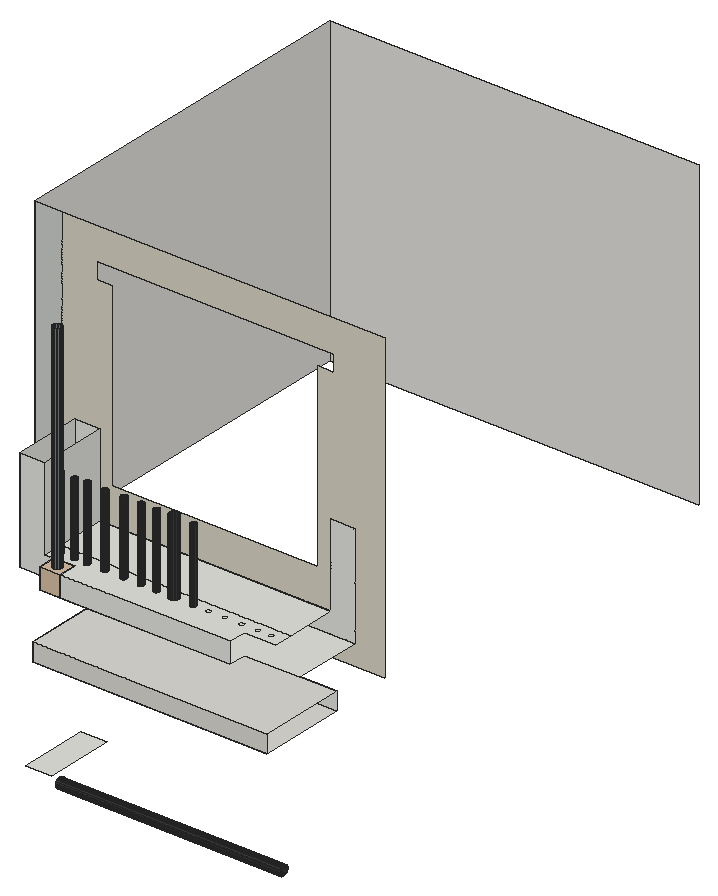
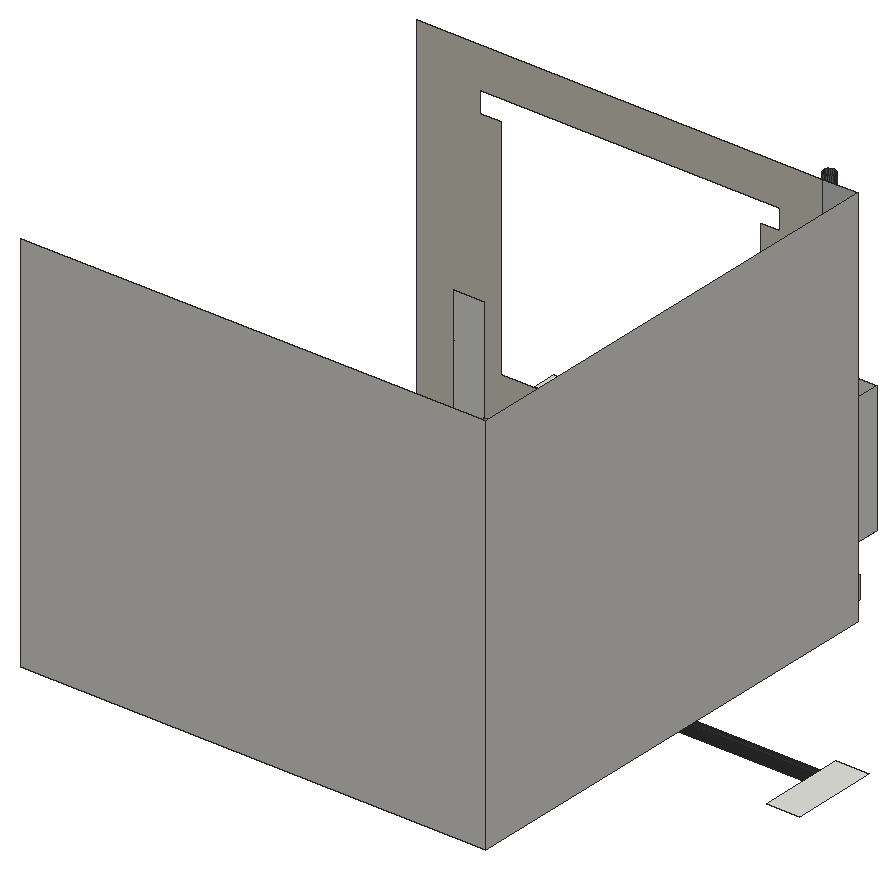
# SketchUp Ruby script. Lengths in inches.
U = 1.inch
M = Sketchup.active_model
def pt(a) = Geom::Point3d.new(a.map { |v| v * U })
def face(e, loops, mat)
  f = e.add_face(loops[0].map { |a| pt(a) })
  loops[1..].each { |l| e.add_face(l.map { |a| pt(a) }).erase! }
  f.material = f.back_material = mat if mat
  f
end
# faces: each face lists its corners as indices into pts; further lists are holes
def faces(e, pts, list, mat = nil) = list.each { |f| face(e, (f[0].is_a?(Array) ? f : [f]).map { |l| l.map { |i| pts[i] } }, mat) }
# xy, xz, yz: faces in a plane at the given z, y or x. An outline is a flat list of corners, or four numbers for a rectangle; further outlines are holes
def ring(l) = l.size == 4 ? [[l[0], l[1]], [l[2], l[1]], [l[2], l[3]], [l[0], l[3]]] : l.each_slice(2).to_a
def flat(e, list, mat, &to3) = list.each { |f| face(e, (f[0].is_a?(Array) ? f : [f]).map { |l| ring(l).map { |u, v| to3.(u, v) } }, mat) }
def xy(e, z, list, mat = nil) = flat(e, list, mat) { |x, y| [x, y, z] }
def xz(e, y, list, mat = nil) = flat(e, list, mat) { |x, z| [x, y, z] }
def yz(e, x, list, mat = nil) = flat(e, list, mat) { |y, z| [x, y, z] }
def lines(e, pts, list) = list.each { |a, b| e.add_line(pt(pts[a]), pt(pts[b])) }
# prism: a flat outline (further loops are holes) pulled along v
def prism(e, loops, v, mat = nil)
  f = face(e, loops, mat); d = Geom::Vector3d.new(v.map { |x| x * U })
  f.pushpull(f.normal.samedirection?(d) ? d.length : -d.length)
end
def box(e, o, s, mat = nil) = prism(e, [[o, [o[0] + s[0], o[1], o[2]], [o[0] + s[0], o[1] + s[1], o[2]], [o[0], o[1] + s[1], o[2]]]], [0, 0, s[2]], mat)
def at(x, y, z, deg = 0) = Geom::Transformation.translation(pt([x, y, z])) * Geom::Transformation.rotation(ORIGIN, Z_AXIS, deg.degrees)
def axes(o, x, y, z) = Geom::Transformation.new([*x, 0, *y, 0, *z, 0, *pt(o).to_a, 1])
def part(name) = M.definitions.add(name)
# library, detail: a bought-in or finely detailed component or shape, given as its bounding box
def library(name, o, s) = part(name).tap { |d| box(d.entities, o, s) }
def detail(e, o, s) = box(e.add_group.entities, o, s)
def put(e, d, t, mat = nil) = e.add_instance(d, t).tap { |i| i.material = mat if mat }
def group(e, t, mat = nil) = e.add_group.tap { |g| g.transformation = t; g.material = mat if mat }.entities
root = M.entities
M.materials.add("[Basic Tile]").color = [203, 206, 202]
M.materials.add("[Color M07]").color = [58, 58, 58]
M.materials.add("[Formica Graystone]1").color = [216, 212, 196]
M.materials.add("[Formica Laminate Light]").color = [213, 189, 164]
M.materials.add("[Formica Speckled Grey]").color = [112, 125, 132]
M.materials.add("[Quartz Light Brown]").color = [199, 184, 152]
M.materials.add("[Terrazzo Tile Accent]").color = [224, 221, 217]
M.materials.add("[Terrazzo Tile Light]").color = [219, 217, 210]
xy(root,298.58,[[85.8,91.86,86.02,91.89,86.24,91.97,86.42,92.11,86.56,92.29,86.64,92.5,86.67,92.73,86.64,92.96,86.56,93.17,86.42,93.35,86.24,93.49,86.02,93.58,85.8,93.61,85.57,93.58,85.36,93.49,85.18,93.35,85.04,93.17,84.95,92.96,84.92,92.73,84.95,92.5,85.04,92.29,85.18,92.11,85.36,91.97,85.57,91.89]])
xy(root,298.77,[[73.9,91.87,74.08,91.89,74.25,91.96,74.39,92.07,74.5,92.21,74.57,92.38,74.59,92.56,74.57,92.73,74.5,92.9,74.39,93.04,74.25,93.15,74.08,93.22,73.9,93.24,73.73,93.22,73.5625,93.15,73.42,93.04,73.31,92.9,73.24,92.73,73.22,92.56,73.24,92.38,73.31,92.21,73.42,92.07,73.5625,91.96,73.73,91.89]])
xy(root,299.33,[[67.78,91.87,67.96,91.89,68.125,91.96,68.27,92.07,68.375,92.21,68.44,92.38,68.47,92.56,68.44,92.73,68.375,92.9,68.27,93.04,68.125,93.15,67.96,93.22,67.78,93.24,67.6,93.22,67.4375,93.15,67.29,93.04,67.18,92.9,67.12,92.73,67.09,92.56,67.12,92.38,67.18,92.21,67.29,92.07,67.4375,91.96,67.6,91.89]])
xy(root,299.71,[[50.09,91.87,50.27,91.89,50.4375,91.96,50.58,92.07,50.6875,92.21,50.76,92.38,50.78,92.56,50.76,92.73,50.6875,92.9,50.58,93.04,50.4375,93.15,50.27,93.22,50.09,93.24,49.91,93.22,49.75,93.15,49.61,93.04,49.5,92.9,49.43,92.73,49.4,92.56,49.43,92.38,49.5,92.21,49.61,92.07,49.75,91.96,49.91,91.89]])
xy(root,299.74,[[55.47,91.87,55.64,91.89,55.8125,91.96,55.95,92.07,56.0625,92.21,56.13,92.38,56.15,92.56,56.13,92.73,56.0625,92.9,55.95,93.04,55.8125,93.15,55.64,93.22,55.47,93.24,55.29,93.22,55.125,93.15,54.98,93.04,54.87,92.9,54.8,92.73,54.78,92.56,54.8,92.38,54.87,92.21,54.98,92.07,55.125,91.96,55.29,91.89],[61.72,91.87,61.89,91.89,62.0625,91.96,62.2,92.07,62.3125,92.21,62.38,92.38,62.4,92.56,62.38,92.73,62.3125,92.9,62.2,93.04,62.0625,93.15,61.89,93.22,61.72,93.24,61.54,93.22,61.375,93.15,61.23,93.04,61.12,92.9,61.05,92.73,61.03,92.56,61.05,92.38,61.12,92.21,61.23,92.07,61.375,91.96,61.54,91.89],[80.03,91.87,80.21,91.89,80.375,91.96,80.52,92.07,80.625,92.21,80.69,92.38,80.72,92.56,80.69,92.73,80.625,92.9,80.52,93.04,80.375,93.15,80.21,93.22,80.03,93.24,79.85,93.22,79.6875,93.15,79.54,93.04,79.43,92.9,79.37,92.73,79.34,92.56,79.37,92.38,79.43,92.21,79.54,92.07,79.6875,91.96,79.85,91.89],[90.97,91.87,91.14,91.89,91.3125,91.96,91.45,92.07,91.5625,92.21,91.63,92.38,91.65,92.56,91.63,92.73,91.5625,92.9,91.45,93.04,91.3125,93.15,91.14,93.22,90.97,93.24,90.79,93.22,90.625,93.15,90.48,93.04,90.37,92.9,90.3,92.73,90.28,92.56,90.3,92.38,90.37,92.21,90.48,92.07,90.625,91.96,90.79,91.89]])
xy(root,302.83,[[37.87,89.73,47.16,114.1]])
xy(root,338.67,[[51.12,107.85,119.37,114.1]],"[Quartz Light Brown]")
xy(root,339.99,[[51.12,107.85,119.37,109.1],[51.12,109.1,119.37,114.1]])
xy(root,341.31,[[51.12,109.1,119.37,114.1]])
xy(root,341.31,[[[45.36,83.35,45.36,114.1,51.12,114.1,51.12,109.1,119.37,109.1,119.37,114.1,128.55,114.1,128.55,83.35],[120.4,84.29,120.93,84.36,121.43,84.57,121.86,84.89,122.18,85.32,122.39,85.82,122.46,86.35,122.39,86.89,122.18,87.38,121.86,87.8125,121.43,88.14,120.93,88.35,120.4,88.42,119.86,88.35,119.37,88.14,118.9375,87.8125,118.61,87.38,118.41,86.89,118.33,86.35,118.41,85.82,118.61,85.32,118.9375,84.89,119.37,84.57,119.86,84.36],[54.33,84.29,54.87,84.36,55.37,84.57,55.79,84.89,56.12,85.32,56.33,85.82,56.4,86.35,56.33,86.89,56.12,87.38,55.79,87.8125,55.37,88.14,54.87,88.35,54.33,88.42,53.8,88.35,53.3,88.14,52.875,87.8125,52.55,87.38,52.34,86.89,52.27,86.35,52.34,85.82,52.55,85.32,52.875,84.89,53.3,84.57,53.8,84.36]]],"[Terrazzo Tile Light]")
xy(root,347.68,[[45.36,83.35,128.55,114.1]],"[Terrazzo Tile Light]")
xy(root,365.02,[[55.11,83.42,55.11,89.73,35.74,89.73,35.74,114.1,135.17,114.1,135.17,89.73,115.36,89.73,115.36,83.42]])
xy(root,365.02,[[47.86,83.42,55.11,89.73]],"[Formica Laminate Light]")
xy(root,372.27,[[[55.11,83.42,115.36,83.42,115.36,89.73,126.56,89.73,126.56,96.33,44.74,96.33,44.74,89.73,55.11,89.73],[87.78,91.42,87.36,91.47,86.97,91.63,86.63,91.89,86.375,92.23,86.21,92.62,86.16,93.04,86.21,93.46,86.375,93.85,86.63,94.19,86.97,94.45,87.36,94.61,87.78,94.67,88.2,94.61,88.59,94.45,88.93,94.19,89.1875,93.85,89.35,93.46,89.41,93.04,89.35,92.62,89.1875,92.23,88.93,91.89,88.59,91.63,88.2,91.47],[94.65,92.0625,94.39,92.1,94.15,92.2,93.94,92.35,93.78,92.5625,93.68,92.8,93.65,93.0625,93.68,93.32,93.78,93.5625,93.94,93.77,94.15,93.93,94.39,94.03,94.65,94.0625,94.91,94.03,95.15,93.93,95.36,93.77,95.52,93.5625,95.62,93.32,95.65,93.0625,95.62,92.8,95.52,92.5625,95.36,92.35,95.15,92.2,94.91,92.1],[122.21,92.0625,121.95,92.1,121.71,92.2,121.5,92.35,121.35,92.5625,121.25,92.8,121.21,93.0625,121.25,93.32,121.35,93.5625,121.5,93.77,121.71,93.93,121.95,94.03,122.21,94.0625,122.47,94.03,122.71,93.93,122.92,93.77,123.08,93.5625,123.18,93.32,123.21,93.0625,123.18,92.8,123.08,92.5625,122.92,92.35,122.71,92.2,122.47,92.1],[100.02,92.0625,99.77,92.1,99.52,92.2,99.32,92.35,99.16,92.5625,99.06,92.8,99.02,93.0625,99.06,93.32,99.16,93.5625,99.32,93.77,99.52,93.93,99.77,94.03,100.02,94.0625,100.28,94.03,100.52,93.93,100.73,93.77,100.89,93.5625,100.99,93.32,101.02,93.0625,100.99,92.8,100.89,92.5625,100.73,92.35,100.52,92.2,100.28,92.1],[117.4,92.0625,117.14,92.1,116.9,92.2,116.69,92.35,116.53,92.5625,116.43,92.8,116.4,93.0625,116.43,93.32,116.53,93.5625,116.69,93.77,116.9,93.93,117.14,94.03,117.4,94.0625,117.66,94.03,117.9,93.93,118.11,93.77,118.27,93.5625,118.37,93.32,118.4,93.0625,118.37,92.8,118.27,92.5625,118.11,92.35,117.9,92.2,117.66,92.1],[105.71,92.0625,105.45,92.1,105.21,92.2,105,92.35,104.85,92.5625,104.75,92.8,104.71,93.0625,104.75,93.32,104.85,93.5625,105,93.77,105.21,93.93,105.45,94.03,105.71,94.0625,105.97,94.03,106.21,93.93,106.42,93.77,106.58,93.5625,106.68,93.32,106.71,93.0625,106.68,92.8,106.58,92.5625,106.42,92.35,106.21,92.2,105.97,92.1],[111.77,92.0625,111.52,92.1,111.27,92.2,111.07,92.35,110.91,92.5625,110.81,92.8,110.77,93.0625,110.81,93.32,110.91,93.5625,111.07,93.77,111.27,93.93,111.52,94.03,111.77,94.0625,112.03,94.03,112.27,93.93,112.48,93.77,112.64,93.5625,112.74,93.32,112.77,93.0625,112.74,92.8,112.64,92.5625,112.48,92.35,112.27,92.2,112.03,92.1],[47.34,92.0625,47.08,92.1,46.84,92.2,46.63,92.35,46.47,92.5625,46.37,92.8,46.34,93.0625,46.37,93.32,46.47,93.5625,46.63,93.77,46.84,93.93,47.08,94.03,47.34,94.0625,47.6,94.03,47.84,93.93,48.04,93.77,48.2,93.5625,48.3,93.32,48.34,93.0625,48.3,92.8,48.2,92.5625,48.04,92.35,47.84,92.2,47.6,92.1],[81.59,92.0625,81.33,92.1,81.09,92.2,80.88,92.35,80.72,92.5625,80.62,92.8,80.59,93.0625,80.62,93.32,80.72,93.5625,80.88,93.77,81.09,93.93,81.33,94.03,81.59,94.0625,81.85,94.03,82.09,93.93,82.29,93.77,82.45,93.5625,82.55,93.32,82.59,93.0625,82.55,92.8,82.45,92.5625,82.29,92.35,82.09,92.2,81.85,92.1],[52.52,92.0625,52.27,92.1,52.02,92.2,51.82,92.35,51.66,92.5625,51.56,92.8,51.52,93.0625,51.56,93.32,51.66,93.5625,51.82,93.77,52.02,93.93,52.27,94.03,52.52,94.0625,52.78,94.03,53.02,93.93,53.23,93.77,53.39,93.5625,53.49,93.32,53.52,93.0625,53.49,92.8,53.39,92.5625,53.23,92.35,53.02,92.2,52.78,92.1],[76.09,92.0625,75.83,92.1,75.59,92.2,75.38,92.35,75.22,92.5625,75.12,92.8,75.09,93.0625,75.12,93.32,75.22,93.5625,75.38,93.77,75.59,93.93,75.83,94.03,76.09,94.0625,76.35,94.03,76.59,93.93,76.79,93.77,76.95,93.5625,77.05,93.32,77.09,93.0625,77.05,92.8,76.95,92.5625,76.79,92.35,76.59,92.2,76.35,92.1],[56.96,92.0625,56.7,92.1,56.46,92.2,56.25,92.35,56.1,92.5625,56,92.8,55.96,93.0625,56,93.32,56.1,93.5625,56.25,93.77,56.46,93.93,56.7,94.03,56.96,94.0625,57.22,94.03,57.46,93.93,57.67,93.77,57.83,93.5625,57.93,93.32,57.96,93.0625,57.93,92.8,57.83,92.5625,57.67,92.35,57.46,92.2,57.22,92.1],[69.96,92.0625,69.7,92.1,69.46,92.2,69.25,92.35,69.1,92.5625,69,92.8,68.96,93.0625,69,93.32,69.1,93.5625,69.25,93.77,69.46,93.93,69.7,94.03,69.96,94.0625,70.22,94.03,70.46,93.93,70.67,93.77,70.83,93.5625,70.93,93.32,70.96,93.0625,70.93,92.8,70.83,92.5625,70.67,92.35,70.46,92.2,70.22,92.1],[63.21,92.0625,62.95,92.1,62.71,92.2,62.5,92.35,62.35,92.5625,62.25,92.8,62.21,93.0625,62.25,93.32,62.35,93.5625,62.5,93.77,62.71,93.93,62.95,94.03,63.21,94.0625,63.47,94.03,63.71,93.93,63.92,93.77,64.08,93.5625,64.18,93.32,64.21,93.0625,64.18,92.8,64.08,92.5625,63.92,92.35,63.71,92.2,63.47,92.1]],[51.5,85,51.08,85.06,50.6875,85.22,50.35,85.48,50.09,85.82,49.93,86.21,49.875,86.63,49.93,87.05,50.09,87.44,50.35,87.78,50.6875,88.04,51.08,88.2,51.5,88.25,51.92,88.2,52.3125,88.04,52.65,87.78,52.91,87.44,53.07,87.05,53.125,86.63,53.07,86.21,52.91,85.82,52.65,85.48,52.3125,85.22,51.92,85.06],[87.78,91.42,87.36,91.47,86.97,91.63,86.63,91.89,86.375,92.23,86.21,92.62,86.16,93.04,86.21,93.46,86.375,93.85,86.63,94.19,86.97,94.45,87.36,94.61,87.78,94.67,88.2,94.61,88.59,94.45,88.93,94.19,89.1875,93.85,89.35,93.46,89.41,93.04,89.35,92.62,89.1875,92.23,88.93,91.89,88.59,91.63,88.2,91.47],[47.34,92.0625,47.08,92.1,46.84,92.2,46.63,92.35,46.47,92.5625,46.37,92.8,46.34,93.0625,46.37,93.32,46.47,93.5625,46.63,93.77,46.84,93.93,47.08,94.03,47.34,94.0625,47.6,94.03,47.84,93.93,48.04,93.77,48.2,93.5625,48.3,93.32,48.34,93.0625,48.3,92.8,48.2,92.5625,48.04,92.35,47.84,92.2,47.6,92.1],[52.52,92.0625,52.27,92.1,52.02,92.2,51.82,92.35,51.66,92.5625,51.56,92.8,51.52,93.0625,51.56,93.32,51.66,93.5625,51.82,93.77,52.02,93.93,52.27,94.03,52.52,94.0625,52.78,94.03,53.02,93.93,53.23,93.77,53.39,93.5625,53.49,93.32,53.52,93.0625,53.49,92.8,53.39,92.5625,53.23,92.35,53.02,92.2,52.78,92.1],
  [56.96,92.0625,56.7,92.1,56.46,92.2,56.25,92.35,56.1,92.5625,56,92.8,55.96,93.0625,56,93.32,56.1,93.5625,56.25,93.77,56.46,93.93,56.7,94.03,56.96,94.0625,57.22,94.03,57.46,93.93,57.67,93.77,57.83,93.5625,57.93,93.32,57.96,93.0625,57.93,92.8,57.83,92.5625,57.67,92.35,57.46,92.2,57.22,92.1],[63.21,92.0625,62.95,92.1,62.71,92.2,62.5,92.35,62.35,92.5625,62.25,92.8,62.21,93.0625,62.25,93.32,62.35,93.5625,62.5,93.77,62.71,93.93,62.95,94.03,63.21,94.0625,63.47,94.03,63.71,93.93,63.92,93.77,64.08,93.5625,64.18,93.32,64.21,93.0625,64.18,92.8,64.08,92.5625,63.92,92.35,63.71,92.2,63.47,92.1],[69.96,92.0625,69.7,92.1,69.46,92.2,69.25,92.35,69.1,92.5625,69,92.8,68.96,93.0625,69,93.32,69.1,93.5625,69.25,93.77,69.46,93.93,69.7,94.03,69.96,94.0625,70.22,94.03,70.46,93.93,70.67,93.77,70.83,93.5625,70.93,93.32,70.96,93.0625,70.93,92.8,70.83,92.5625,70.67,92.35,70.46,92.2,70.22,92.1],[76.09,92.0625,75.83,92.1,75.59,92.2,75.38,92.35,75.22,92.5625,75.12,92.8,75.09,93.0625,75.12,93.32,75.22,93.5625,75.38,93.77,75.59,93.93,75.83,94.03,76.09,94.0625,76.35,94.03,76.59,93.93,76.79,93.77,76.95,93.5625,77.05,93.32,77.09,93.0625,77.05,92.8,76.95,92.5625,76.79,92.35,76.59,92.2,76.35,92.1],[81.59,92.0625,81.33,92.1,81.09,92.2,80.88,92.35,80.72,92.5625,80.62,92.8,80.59,93.0625,80.62,93.32,80.72,93.5625,80.88,93.77,81.09,93.93,81.33,94.03,81.59,94.0625,81.85,94.03,82.09,93.93,82.29,93.77,82.45,93.5625,82.55,93.32,82.59,93.0625,82.55,92.8,82.45,92.5625,82.29,92.35,82.09,92.2,81.85,92.1],
  [94.65,92.0625,94.39,92.1,94.15,92.2,93.94,92.35,93.78,92.5625,93.68,92.8,93.65,93.0625,93.68,93.32,93.78,93.5625,93.94,93.77,94.15,93.93,94.39,94.03,94.65,94.0625,94.91,94.03,95.15,93.93,95.36,93.77,95.52,93.5625,95.62,93.32,95.65,93.0625,95.62,92.8,95.52,92.5625,95.36,92.35,95.15,92.2,94.91,92.1],[44.74,96.33,126.56,114.1]])
xy(root,372.27,[[[47.86,83.42,55.11,89.73],[51.5,85,51.08,85.06,50.6875,85.22,50.35,85.48,50.09,85.82,49.93,86.21,49.875,86.63,49.93,87.05,50.09,87.44,50.35,87.78,50.6875,88.04,51.08,88.2,51.5,88.25,51.92,88.2,52.3125,88.04,52.65,87.78,52.91,87.44,53.07,87.05,53.125,86.63,53.07,86.21,52.91,85.82,52.65,85.48,52.3125,85.22,51.92,85.06]]],"[Formica Laminate Light]")
xz(root,83.35,[[45.36,341.31,128.55,347.68]],"[Terrazzo Tile Light]")
xz(root,83.42,[[55.11,365.02,115.36,372.27]])
xz(root,83.42,[[47.86,365.02,55.11,372.27]],"[Formica Laminate Light]")
xz(root,89.73,[[35.74,365.02,47.86,365.02,47.86,372.27,44.74,372.27,44.74,401.52,35.74,401.52],[47.86,365.02,55.11,372.27]])
xz(root,107.85,[[51.12,338.67,119.37,339.99]],"[Quartz Light Brown]")
xz(root,109.1,[[51.12,339.99,119.37,341.31]],"[Quartz Light Brown]")
xz(root,114.1,[[51.12,338.67,119.37,339.99],[51.12,339.99,119.37,341.31],[45.36,341.31,128.55,347.68],[35.74,365.02,35.74,401.52,44.74,401.52,44.74,372.27,126.56,372.27,126.56,401.52,135.17,401.52,135.17,365.02]])
xz(root,114.1,[[21.57,357.6875,31.29,465.6875]],"[Basic Tile]")
xz(root,114.1,[[[31.29,357.6875,145.58,465.6875],[48.8,384.74,48.8,448.43,43.4,448.43,43.4,454.37,127.71,454.37,127.71,448.43,121.8,448.43,121.8,384.74],[35.74,365.02,35.74,401.52,44.74,401.52,44.74,372.27,126.56,372.27,126.56,401.52,135.17,401.52,135.17,365.02]]],"[Formica Graystone]1")
xz(root,244.83,[[21.57,357.6875,152.39,465.6875]],"[Terrazzo Tile Accent]")
yz(root,21.57,[[114.1,357.6875,244.83,465.6875]],"[Terrazzo Tile Accent]")
yz(root,35.74,[[89.73,365.02,114.1,401.52]])
yz(root,44.74,[[[89.73,372.27,114.1,401.52],[93.49,396.95,93.16,396.99,92.86,397.12,92.6,397.32,92.4,397.58,92.28,397.88,92.24,398.2,92.28,398.52,92.4,398.83,92.6,399.09,92.86,399.28,93.16,399.41,93.49,399.45,93.81,399.41,94.11,399.28,94.37,399.09,94.57,398.83,94.69,398.52,94.74,398.2,94.69,397.88,94.57,397.58,94.37,397.32,94.11,397.12,93.81,396.99],[93.62,385.75,93.3125,385.79,93.03,385.91,92.78,386.1,92.59,386.34,92.47,386.63,92.43,386.9375,92.47,387.25,92.59,387.53,92.78,387.78,93.03,387.97,93.3125,388.09,93.62,388.125,93.93,388.09,94.21,387.97,94.46,387.78,94.65,387.53,94.77,387.25,94.81,386.9375,94.77,386.63,94.65,386.34,94.46,386.1,94.21,385.91,93.93,385.79]]])
yz(root,45.36,[[83.35,341.31,114.1,347.68]],"[Terrazzo Tile Light]")
yz(root,47.86,[[83.42,365.02,89.73,372.27]],"[Formica Laminate Light]")
yz(root,51.12,[[107.85,338.67,114.1,339.99],[109.1,339.99,114.1,341.31]],"[Quartz Light Brown]")
yz(root,55.11,[[83.42,365.02,89.73,372.27]])
p = [[126.66,92.96,297.54],[126.66,92.51,297.6],[47.16,92.51,297.6],[47.16,92.96,297.54],[126.66,93.42,297.6],[47.16,93.42,297.6],
  [126.66,92.09,297.77],[47.16,92.09,297.77],[126.66,93.84,297.77],[47.16,93.84,297.77],[126.66,91.73,298.05],[47.16,91.73,298.05],
  [126.66,94.2,298.05],[47.16,94.2,298.05],[126.66,91.45,298.41],[47.16,91.45,298.41],[126.66,94.48,298.41],[47.16,94.48,298.41],
  [126.66,91.27,298.84],[47.16,91.27,298.84],[126.66,94.65,298.84],[47.16,94.65,298.84],[126.66,91.21,299.29],[47.16,91.21,299.29],
  [126.66,94.71,299.29],[47.16,94.71,299.29],[126.66,91.27,299.74],[47.16,91.27,299.74],[126.66,94.65,299.74],[47.16,94.65,299.74],
  [126.66,91.45,300.16],[47.16,91.45,300.16],[126.66,94.48,300.16],[47.16,94.48,300.16],[126.66,91.73,300.53],[47.16,91.73,300.53],
  [126.66,94.2,300.53],[47.16,94.2,300.53],[126.66,92.09,300.8],[47.16,92.09,300.8],[126.66,93.84,300.8],[47.16,93.84,300.8],
  [126.66,92.51,300.98],[47.16,92.51,300.98],[126.66,93.42,300.98],[47.16,93.42,300.98],[126.66,92.96,301.04],[47.16,92.96,301.04],
  [51.08,85.06,372.27],[51.5,85,372.27],[51.5,85,448.43],[51.08,85.06,448.43],[51.92,85.06,372.27],[51.92,85.06,448.43],
  [50.6875,85.22,372.27],[50.6875,85.22,448.43],[52.3125,85.22,372.27],[52.3125,85.22,448.43],[50.35,85.48,372.27],[50.35,85.48,448.43],
  [52.65,85.48,372.27],[52.65,85.48,448.43],[50.09,85.82,372.27],[50.09,85.82,448.43],[52.91,85.82,372.27],[52.91,85.82,448.43],
  [49.93,86.21,372.27],[49.93,86.21,448.43],[53.07,86.21,372.27],[53.07,86.21,448.43],[49.875,86.63,372.27],[49.875,86.63,448.43],
  [53.125,86.63,372.27],[53.125,86.63,448.43],[49.93,87.05,372.27],[49.93,87.05,448.43],[53.07,87.05,372.27],[53.07,87.05,448.43],
  [50.09,87.44,372.27],[50.09,87.44,448.43],[52.91,87.44,372.27],[52.91,87.44,448.43],[50.35,87.78,372.27],[50.35,87.78,448.43],
  [52.65,87.78,372.27],[52.65,87.78,448.43],[50.6875,88.04,372.27],[50.6875,88.04,448.43],[52.3125,88.04,372.27],[52.3125,88.04,448.43],
  [51.08,88.2,372.27],[51.08,88.2,448.43],[51.92,88.2,372.27],[51.92,88.2,448.43],[51.5,88.25,372.27],[51.5,88.25,448.43],
  [87.36,91.47,372.27],[87.78,91.42,372.27],[87.78,91.42,398.83],[87.36,91.47,398.83],[88.2,91.47,372.27],[88.2,91.47,398.83],
  [86.97,91.63,372.27],[86.97,91.63,398.83],[88.59,91.63,372.27],[88.59,91.63,398.83],[86.63,91.89,372.27],[86.63,91.89,398.83],
  [88.93,91.89,372.27],[88.93,91.89,398.83],[86.375,92.23,372.27],[86.375,92.23,398.83],[89.1875,92.23,372.27],[89.1875,92.23,398.83],
  [46.84,92.2,372.27],[47.08,92.1,372.27],[47.08,92.1,398.08],[46.84,92.2,398.08],[47.34,92.0625,372.27],[47.34,92.0625,398.08],
  [47.6,92.1,372.27],[47.6,92.1,398.08],[47.84,92.2,372.27],[47.84,92.2,398.08],[52.02,92.2,372.27],[52.27,92.1,372.27],
  [52.27,92.1,397.9],[52.02,92.2,397.9],[52.52,92.0625,372.27],[52.52,92.0625,397.9],[52.78,92.1,372.27],[52.78,92.1,397.9],
  [53.02,92.2,372.27],[53.02,92.2,397.9],[56.46,92.2,372.27],[56.7,92.1,372.27],[56.7,92.1,398.15],[56.46,92.2,398.15],
  [56.96,92.0625,372.27],[56.96,92.0625,398.15],[57.22,92.1,372.27],[57.22,92.1,398.15],[57.46,92.2,372.27],[57.46,92.2,398.15],
  [62.71,92.2,372.27],[62.95,92.1,372.27],[62.95,92.1,397.9],[62.71,92.2,397.9],[63.21,92.0625,372.27],[63.21,92.0625,397.9],
  [63.47,92.1,372.27],[63.47,92.1,397.9],[63.71,92.2,372.27],[63.71,92.2,397.9],[69.46,92.2,372.27],[69.7,92.1,372.27],
  [69.7,92.1,398.15],[69.46,92.2,398.15],[69.96,92.0625,372.27],[69.96,92.0625,398.15],[70.22,92.1,372.27],[70.22,92.1,398.15],
  [70.46,92.2,372.27],[70.46,92.2,398.15],[75.59,92.2,372.27],[75.83,92.1,372.27],[75.83,92.1,398.15],[75.59,92.2,398.15],
  [76.09,92.0625,372.27],[76.09,92.0625,398.15],[76.35,92.1,372.27],[76.35,92.1,398.15],[76.59,92.2,372.27],[76.59,92.2,398.15],
  [81.09,92.2,372.27],[81.33,92.1,372.27],[81.33,92.1,398.08],[81.09,92.2,398.08],[81.59,92.0625,372.27],[81.59,92.0625,398.08],
  [81.85,92.1,372.27],[81.85,92.1,398.08],[82.09,92.2,372.27],[82.09,92.2,398.08],[94.15,92.2,372.27],[94.39,92.1,372.27],
  [94.39,92.1,398.15],[94.15,92.2,398.15],[94.65,92.0625,372.27],[94.65,92.0625,398.15],[94.91,92.1,372.27],[94.91,92.1,398.15],
  [95.15,92.2,372.27],[95.15,92.2,398.15],[46.63,92.35,372.27],[46.63,92.35,398.08],[48.04,92.35,372.27],[48.04,92.35,398.08],
  [51.82,92.35,372.27],[51.82,92.35,397.9],[53.23,92.35,372.27],[53.23,92.35,397.9],[56.25,92.35,372.27],[56.25,92.35,398.15],
  [57.67,92.35,372.27],[57.67,92.35,398.15],[62.5,92.35,372.27],[62.5,92.35,397.9],[63.92,92.35,372.27],[63.92,92.35,397.9],
  [69.25,92.35,372.27],[69.25,92.35,398.15],[70.67,92.35,372.27],[70.67,92.35,398.15],[75.38,92.35,372.27],[75.38,92.35,398.15],
  [76.79,92.35,372.27],[76.79,92.35,398.15],[80.88,92.35,372.27],[80.88,92.35,398.08],[82.29,92.35,372.27],[82.29,92.35,398.08],
  [86.21,92.62,372.27],[86.3,92.4,398.83],[86.21,92.62,398.83],[89.35,92.62,372.27],[89.35,92.62,398.83],[89.26,92.4,398.83],
  [93.94,92.35,372.27],[93.94,92.35,398.15],[95.36,92.35,372.27],[95.36,92.35,398.15],[46.47,92.5625,372.27],[46.47,92.5625,398.08],
  [48.2,92.5625,372.27],[48.2,92.5625,398.08],[51.66,92.5625,372.27],[51.66,92.5625,397.9],[53.39,92.5625,372.27],[53.39,92.5625,397.9],
  [56.1,92.5625,372.27],[56.1,92.5625,398.15],[57.83,92.5625,372.27],[57.83,92.5625,398.15],[62.35,92.5625,372.27],[62.35,92.5625,397.9],
  [64.08,92.5625,372.27],[64.08,92.5625,397.9],[69.1,92.5625,372.27],[69.1,92.5625,398.15],[70.83,92.5625,372.27],[70.83,92.5625,398.15],
  [75.22,92.5625,372.27],[75.22,92.5625,398.15],[76.95,92.5625,372.27],[76.95,92.5625,398.15],[80.72,92.5625,372.27],[80.72,92.5625,398.08],
  [82.45,92.5625,372.27],[82.45,92.5625,398.08],[93.78,92.5625,372.27],[93.78,92.5625,398.15],[95.52,92.5625,372.27],[95.52,92.5625,398.15],
  [46.37,92.8,372.27],[46.37,92.8,398.08],[48.3,92.8,372.27],[48.3,92.8,398.08],[51.56,92.8,372.27],[51.56,92.8,397.9],
  [53.49,92.8,372.27],[53.49,92.8,397.9],[56,92.8,372.27],[56,92.8,398.15],[57.93,92.8,372.27],[57.93,92.8,398.15],
  [62.25,92.8,372.27],[62.25,92.8,397.9],[64.18,92.8,372.27],[64.18,92.8,397.9],[69,92.8,372.27],[69,92.8,398.15],
  [70.93,92.8,372.27],[70.93,92.8,398.15],[75.12,92.8,372.27],[75.12,92.8,398.15],[77.05,92.8,372.27],[77.05,92.8,398.15],
  [80.62,92.8,372.27],[80.62,92.8,398.08],[82.55,92.8,372.27],[82.55,92.8,398.08],[86.16,93.04,372.27],[86.16,93.04,398.83],
  [89.41,93.04,372.27],[89.41,93.04,398.83],[93.68,92.8,372.27],[93.68,92.8,398.15],[95.62,92.8,372.27],[95.62,92.8,398.15],
  [46.34,93.0625,372.27],[46.34,93.0625,398.08],[48.34,93.0625,372.27],[48.34,93.0625,398.08],[51.52,93.0625,372.27],[51.52,93.0625,397.9],
  [53.52,93.0625,372.27],[53.52,93.0625,397.9],[55.96,93.0625,372.27],[55.96,93.0625,398.15],[57.96,93.0625,372.27],[57.96,93.0625,398.15],
  [62.21,93.0625,372.27],[62.21,93.0625,397.9],[64.21,93.0625,372.27],[64.21,93.0625,397.9],[68.96,93.0625,372.27],[68.96,93.0625,398.15],
  [70.96,93.0625,372.27],[70.96,93.0625,398.15],[75.09,93.0625,372.27],[75.09,93.0625,398.15],[77.09,93.0625,372.27],[77.09,93.0625,398.15],
  [80.59,93.0625,372.27],[80.59,93.0625,398.08],[82.59,93.0625,372.27],[82.59,93.0625,398.08],[93.65,93.0625,372.27],[93.65,93.0625,398.15],
  [86.21,93.46,372.27],[86.21,93.46,398.83],[89.35,93.46,372.27],[89.35,93.46,398.83],[46.37,93.32,372.27],[46.37,93.32,398.08],
  [48.3,93.32,372.27],[48.3,93.32,398.08],[51.56,93.32,372.27],[51.56,93.32,397.9],[53.49,93.32,372.27],[53.49,93.32,397.9],
  [56,93.32,372.27],[56,93.32,398.15],[57.93,93.32,372.27],[57.93,93.32,398.15],[62.25,93.32,372.27],[62.25,93.32,397.9],
  [64.18,93.32,372.27],[64.18,93.32,397.9],[69,93.32,372.27],[69,93.32,398.15],[70.93,93.32,372.27],[70.93,93.32,398.15],
  [75.12,93.32,372.27],[75.12,93.32,398.15],[77.05,93.32,372.27],[77.05,93.32,398.15],[80.62,93.32,372.27],[80.62,93.32,398.08],
  [82.55,93.32,372.27],[82.55,93.32,398.08],[93.68,93.32,372.27],[93.68,93.32,398.15],[46.47,93.5625,372.27],[46.47,93.5625,398.08],
  [48.2,93.5625,372.27],[48.2,93.5625,398.08],[51.66,93.5625,372.27],[51.66,93.5625,397.9],[53.39,93.5625,372.27],[53.39,93.5625,397.9],
  [56.1,93.5625,372.27],[56.1,93.5625,398.15],[57.83,93.5625,372.27],[57.83,93.5625,398.15],[62.35,93.5625,372.27],[62.35,93.5625,397.9],
  [64.08,93.5625,372.27],[64.08,93.5625,397.9],[69.1,93.5625,372.27],[69.1,93.5625,398.15],[70.83,93.5625,372.27],[70.83,93.5625,398.15],
  [75.22,93.5625,372.27],[75.22,93.5625,398.15],[76.95,93.5625,372.27],[76.95,93.5625,398.15],[80.72,93.5625,372.27],[80.72,93.5625,398.08],
  [82.45,93.5625,372.27],[82.45,93.5625,398.08],[93.78,93.5625,372.27],[93.78,93.5625,398.15],[95.62,93.32,372.27],[95.52,93.5625,372.27],
  [95.52,93.5625,398.15],[95.62,93.32,398.15],[86.375,93.85,372.27],[86.375,93.85,398.83],[89.1875,93.85,372.27],[89.1875,93.85,398.83],
  [46.63,93.77,372.27],[46.63,93.77,398.08],[48.04,93.77,372.27],[48.04,93.77,398.08],[51.82,93.77,372.27],[51.82,93.77,397.9],
  [53.23,93.77,372.27],[53.23,93.77,397.9],[56.25,93.77,372.27],[56.25,93.77,398.15],[57.67,93.77,372.27],[57.67,93.77,398.15],
  [62.5,93.77,372.27],[62.5,93.77,397.9],[63.92,93.77,372.27],[63.92,93.77,397.9],[69.25,93.77,372.27],[69.25,93.77,398.15],
  [70.67,93.77,372.27],[70.67,93.77,398.15],[75.38,93.77,372.27],[75.38,93.77,398.15],[76.79,93.77,372.27],[76.79,93.77,398.15],
  [80.88,93.77,372.27],[80.88,93.77,398.08],[82.29,93.77,372.27],[82.29,93.77,398.08],[93.94,93.77,372.27],[93.94,93.77,398.15],
  [95.36,93.77,372.27],[95.36,93.77,398.15],[46.84,93.93,372.27],[46.84,93.93,398.08],[46.84,93.93,388.09],[46.84,93.93,385.79],
  [47.84,93.93,372.27],[47.84,93.93,385.79],[47.84,93.93,388.09],[47.84,93.93,398.08],[52.02,93.93,372.27],[52.02,93.93,397.9],
  [52.02,93.93,388.09],[52.02,93.93,385.79],[53.02,93.93,372.27],[53.02,93.93,385.79],[53.02,93.93,388.09],[53.02,93.93,397.9],
  [56.46,93.93,372.27],[56.46,93.93,398.15],[56.46,93.93,388.09],[56.46,93.93,385.79],[57.46,93.93,372.27],[57.46,93.93,385.79],
  [57.46,93.93,388.09],[57.46,93.93,398.15],[62.71,93.93,372.27],[62.71,93.93,397.9],[62.71,93.93,388.09],[62.71,93.93,385.79],
  [63.71,93.93,372.27],[63.71,93.93,385.79],[63.71,93.93,388.09],[63.71,93.93,397.9],[69.46,93.93,372.27],[69.46,93.93,398.15],
  [69.46,93.93,388.09],[69.46,93.93,385.79],[70.46,93.93,372.27],[70.46,93.93,385.79],[70.46,93.93,388.09],[70.46,93.93,398.15],
  [75.59,93.93,372.27],[75.59,93.93,398.15],[75.59,93.93,388.09],[75.59,93.93,385.79],[76.59,93.93,372.27],[76.59,93.93,385.79],
  [76.59,93.93,388.09],[76.59,93.93,398.15],[81.09,93.93,372.27],[81.09,93.93,398.08],[81.09,93.93,388.09],[81.09,93.93,385.79],
  [82.09,93.93,372.27],[82.09,93.93,385.79],[82.09,93.93,388.09],[82.09,93.93,398.08],[94.15,93.93,372.27],[94.15,93.93,398.15],
  [94.15,93.93,388.09],[94.15,93.93,385.79],[95.15,93.93,372.27],[95.15,93.93,385.79],[95.15,93.93,388.09],[95.15,93.93,398.15],
  [47.08,94.03,372.27],[47.08,94.03,398.08],[47.6,94.03,372.27],[47.6,94.03,398.08],[52.27,94.03,372.27],[52.27,94.03,397.9],
  [52.78,94.03,372.27],[52.78,94.03,397.9],[56.7,94.03,372.27],[56.7,94.03,398.15],[57.22,94.03,372.27],[57.22,94.03,398.15],
  [62.95,94.03,372.27],[62.95,94.03,397.9],[63.47,94.03,372.27],[63.47,94.03,397.9],[69.7,94.03,372.27],[69.7,94.03,398.15],
  [70.22,94.03,372.27],[70.22,94.03,398.15],[75.83,94.03,372.27],[75.83,94.03,398.15],[76.35,94.03,372.27],[76.35,94.03,398.15],
  [81.33,94.03,372.27],[81.33,94.03,398.08],[81.85,94.03,372.27],[81.85,94.03,398.08],[86.63,94.19,372.27],[86.63,94.19,398.83],
  [88.93,94.19,372.27],[88.93,94.19,398.83],[94.39,94.03,372.27],[94.39,94.03,398.15],[94.91,94.03,372.27],[94.91,94.03,398.15],
  [47.34,94.0625,372.27],[47.34,94.0625,398.08],[52.52,94.0625,372.27],[52.52,94.0625,397.9],[56.96,94.0625,372.27],[56.96,94.0625,398.15],
  [63.21,94.0625,372.27],[63.21,94.0625,397.9],[69.96,94.0625,372.27],[69.96,94.0625,398.15],[76.09,94.0625,372.27],[76.09,94.0625,398.15],
  [81.59,94.0625,372.27],[81.59,94.0625,398.08],[94.65,94.0625,372.27],[94.65,94.0625,398.15],[86.97,94.45,372.27],[86.97,94.45,398.83],
  [88.59,94.45,372.27],[88.59,94.45,398.83],[87.36,94.61,372.27],[87.26,94.57,398.83],[87.36,94.61,398.83],[88.2,94.61,372.27],
  [88.2,94.61,398.83],[88.31,94.57,398.83],[87.78,94.67,372.27],[87.78,94.67,398.83]]
faces(root,p,[[0,1,2,3],[4,0,3,5],[1,6,7,2],[8,4,5,9],[6,10,11,7],[12,8,9,13],[10,14,15,11],[16,12,13,17],
  [14,18,19,15],[20,16,17,21],[18,22,23,19],[24,20,21,25],[22,26,27,23],[28,24,25,29],[26,30,31,27],[32,28,29,33],
  [30,34,35,31],[36,32,33,37],[34,38,39,35],[40,36,37,41],[38,42,43,39],[44,40,41,45],[42,46,47,43],[46,44,45,47],
  [96,97,98,99],[97,100,101,98],[102,96,99,103],[100,104,105,101],[106,102,103,107],[104,108,109,105],[110,106,107,111],[108,112,113,109],
  [114,115,116,117],[115,118,119,116],[118,120,121,119],[120,122,123,121],[124,125,126,127],[125,128,129,126],[128,130,131,129],[130,132,133,131],
  [134,135,136,137],[135,138,139,136],[138,140,141,139],[140,142,143,141],[144,145,146,147],[145,148,149,146],[148,150,151,149],[150,152,153,151],
  [154,155,156,157],[155,158,159,156],[158,160,161,159],[160,162,163,161],[164,165,166,167],[165,168,169,166],[168,170,171,169],[170,172,173,171],
  [174,175,176,177],[175,178,179,176],[178,180,181,179],[180,182,183,181],[184,185,186,187],[185,188,189,186],[188,190,191,189],[190,192,193,191],
  [194,114,117,195],[122,196,197,123],[198,124,127,199],[132,200,201,133],[202,134,137,203],[142,204,205,143],[206,144,147,207],[152,208,209,153],
  [210,154,157,211],[162,212,213,163],[214,164,167,215],[172,216,217,173],[218,174,177,219],[182,220,221,183],[222,110,111,223,224],[112,225,226,227,113],
  [228,184,187,229],[192,230,231,193],[232,194,195,233],[196,234,235,197],[236,198,199,237],[200,238,239,201],[240,202,203,241],[204,242,243,205],
  [244,206,207,245],[208,246,247,209],[248,210,211,249],[212,250,251,213],[252,214,215,253],[216,254,255,217],[256,218,219,257],[220,258,259,221],
  [260,228,229,261],[230,262,263,231],[264,232,233,265],[234,266,267,235],[268,236,237,269],[238,270,271,239],[272,240,241,273],[242,274,275,243],
  [276,244,245,277],[246,278,279,247],[280,248,249,281],[250,282,283,251],[284,252,253,285],[254,286,287,255],[288,256,257,289],[258,290,291,259],
  [292,222,224,293],[225,294,295,226],[296,260,261,297],[262,298,299,263],[300,264,265,301],[266,302,303,267],[304,268,269,305],[270,306,307,271],
  [308,272,273,309],[274,310,311,275],[312,276,277,313],[278,314,315,279],[316,280,281,317],[282,318,319,283],[320,284,285,321],[286,322,323,287],
  [324,288,289,325],[290,326,327,291],[328,296,297,329],[330,292,293,331],[294,332,333,295],[334,300,301,335],[302,336,337,303],[338,304,305,339],
  [306,340,341,307],[342,308,309,343],[310,344,345,311],[346,312,313,347],[314,348,349,315],[350,316,317,351],[318,352,353,319],[354,320,321,355],
  [322,356,357,323],[358,324,325,359],[326,360,361,327],[362,328,329,363],[364,334,335,365],[336,366,367,337],[368,338,339,369],[340,370,371,341],
  [372,342,343,373],[344,374,375,345],[376,346,347,377],[348,378,379,349],[380,350,351,381],[352,382,383,353],[384,354,355,385],[356,386,387,357],
  [388,358,359,389],[360,390,391,361],[392,362,363,393],[394,395,396,397],[398,330,331,399],[332,400,401,333],[402,364,365,403],[366,404,405,367],
  [406,368,369,407],[370,408,409,371],[410,372,373,411],[374,412,413,375],[414,376,377,415],[378,416,417,379],[418,380,381,419],[382,420,421,383],
  [422,384,385,423],[386,424,425,387],[426,388,389,427],[390,428,429,391],[430,392,393,431],[395,432,433,396],[434,402,403,435,436,437],[404,438,439,440,441,405],
  [442,406,407,443,444,445],[408,446,447,448,449,409],[450,410,411,451,452,453],[412,454,455,456,457,413],[458,414,415,459,460,461],[416,462,463,464,465,417],[466,418,419,467,468,469],[420,470,471,472,473,421],
  [474,422,423,475,476,477],[424,478,479,480,481,425],[482,426,427,483,484,485],[428,486,487,488,489,429],[490,430,431,491,492,493],[432,494,495,496,497,433],[498,434,437,436,435,499],[438,500,501,441,440,439],
  [502,442,445,444,443,503],[446,504,505,449,448,447],[506,450,453,452,451,507],[454,508,509,457,456,455],[510,458,461,460,459,511],[462,512,513,465,464,463],[514,466,469,468,467,515],[470,516,517,473,472,471],
  [518,474,477,476,475,519],[478,520,521,481,480,479],[522,482,485,484,483,523],[486,524,525,489,488,487],[526,398,399,527],[400,528,529,401],[530,490,493,492,491,531],[494,532,533,497,496,495],
  [534,498,499,535],[500,534,535,501],[536,502,503,537],[504,536,537,505],[538,506,507,539],[508,538,539,509],[540,510,511,541],[512,540,541,513],
  [542,514,515,543],[516,542,543,517],[544,518,519,545],[520,544,545,521],[546,522,523,547],[524,546,547,525],[548,530,531,549],[532,548,549,533],
  [550,526,527,551],[528,552,553,529],[554,550,551,555,556],[552,557,558,559,553],[560,554,556,561],[557,560,561,558]],"[Color M07]")
faces(root,p,[[48,49,50,51],[49,52,53,50],[54,48,51,55],[52,56,57,53],[58,54,55,59],[56,60,61,57],[62,58,59,63],[60,64,65,61],
  [66,62,63,67],[64,68,69,65],[70,66,67,71],[68,72,73,69],[74,70,71,75],[72,76,77,73],[78,74,75,79],[76,80,81,77],
  [82,78,79,83],[80,84,85,81],[86,82,83,87],[84,88,89,85],[90,86,87,91],[88,92,93,89],[94,90,91,95],[92,94,95,93]],"[Formica Speckled Grey]")
